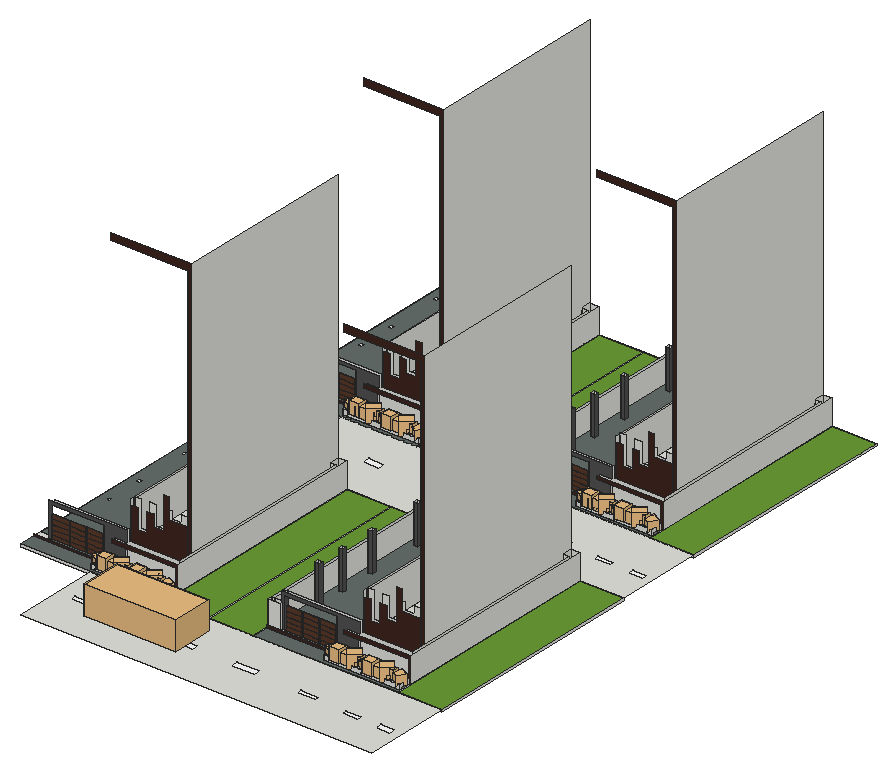
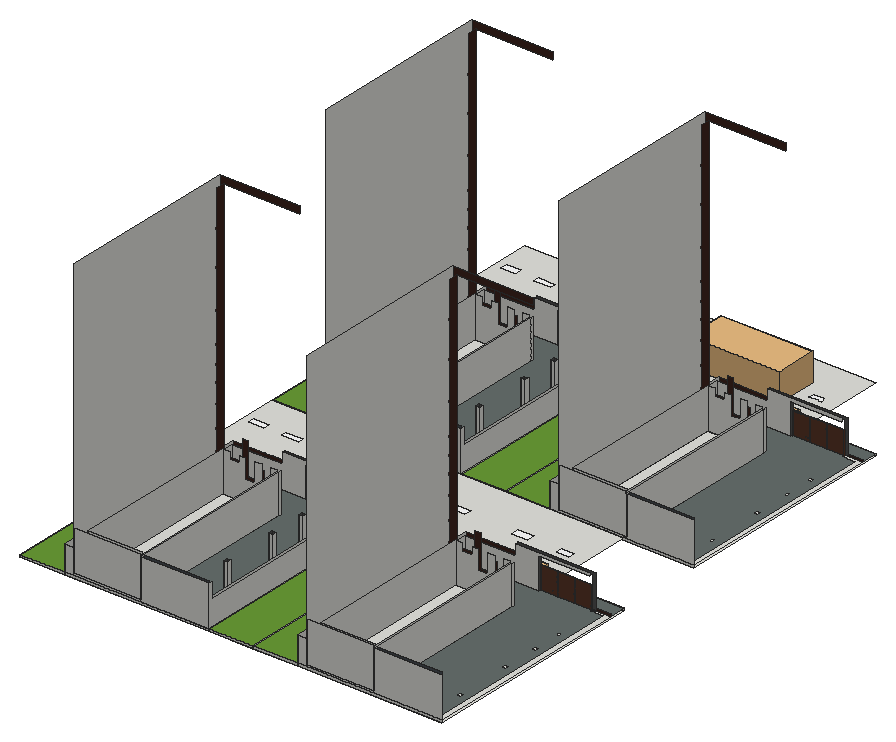
# SketchUp Ruby script. Lengths in inches.
U = 1.inch
M = Sketchup.active_model
def pt(a) = Geom::Point3d.new(a.map { |v| v * U })
def face(e, loops, mat)
  f = e.add_face(loops[0].map { |a| pt(a) })
  loops[1..].each { |l| e.add_face(l.map { |a| pt(a) }).erase! }
  f.material = f.back_material = mat if mat
  f
end
# faces: each face lists its corners as indices into pts; further lists are holes
def faces(e, pts, list, mat = nil) = list.each { |f| face(e, (f[0].is_a?(Array) ? f : [f]).map { |l| l.map { |i| pts[i] } }, mat) }
# xy, xz, yz: faces in a plane at the given z, y or x. An outline is a flat list of corners, or four numbers for a rectangle; further outlines are holes
def ring(l) = l.size == 4 ? [[l[0], l[1]], [l[2], l[1]], [l[2], l[3]], [l[0], l[3]]] : l.each_slice(2).to_a
def flat(e, list, mat, &to3) = list.each { |f| face(e, (f[0].is_a?(Array) ? f : [f]).map { |l| ring(l).map { |u, v| to3.(u, v) } }, mat) }
def xy(e, z, list, mat = nil) = flat(e, list, mat) { |x, y| [x, y, z] }
def xz(e, y, list, mat = nil) = flat(e, list, mat) { |x, z| [x, y, z] }
def yz(e, x, list, mat = nil) = flat(e, list, mat) { |y, z| [x, y, z] }
def lines(e, pts, list) = list.each { |a, b| e.add_line(pt(pts[a]), pt(pts[b])) }
# prism: a flat outline (further loops are holes) pulled along v
def prism(e, loops, v, mat = nil)
  f = face(e, loops, mat); d = Geom::Vector3d.new(v.map { |x| x * U })
  f.pushpull(f.normal.samedirection?(d) ? d.length : -d.length)
end
def box(e, o, s, mat = nil) = prism(e, [[o, [o[0] + s[0], o[1], o[2]], [o[0] + s[0], o[1] + s[1], o[2]], [o[0], o[1] + s[1], o[2]]]], [0, 0, s[2]], mat)
def at(x, y, z, deg = 0) = Geom::Transformation.translation(pt([x, y, z])) * Geom::Transformation.rotation(ORIGIN, Z_AXIS, deg.degrees)
def axes(o, x, y, z) = Geom::Transformation.new([*x, 0, *y, 0, *z, 0, *pt(o).to_a, 1])
def part(name) = M.definitions.add(name)
# library, detail: a bought-in or finely detailed component or shape, given as its bounding box
def library(name, o, s) = part(name).tap { |d| box(d.entities, o, s) }
def detail(e, o, s) = box(e.add_group.entities, o, s)
def put(e, d, t, mat = nil) = e.add_instance(d, t).tap { |i| i.material = mat if mat }
def group(e, t, mat = nil) = e.add_group.tap { |g| g.transformation = t; g.material = mat if mat }.entities
root = M.entities
M.materials.add("Color_").color = [255, 255, 255]
M.materials.add("Material__1").color = [95, 70, 46]
M.materials.add("[0043_SaddleBrown]").color = [63, 38, 31]
M.materials.add("[0135_DarkGray]").color = [81, 81, 81]
M.materials.add("[Color L16]").color = [51, 38, 20]
M.materials.add("[Formica Blue]").color = [73, 80, 86]
M.materials.add("[Grass Dark Green]").color = [105, 155, 54]
M.materials.add("[Slate]").color = [102, 110, 108]
M.materials.add("[Wood Veneer 01]").color = [89, 56, 41]
c1 = part("Grupo\#4")
xy(c1.entities,0,[[0,0,0,3.15,255.91,3.15,255.91,0,171.65,0,171.65,1.57,171.26,1.57,171.26,0,86.22,0,86.22,1.57,85.83,1.57,85.83,0]],"[Wood Veneer 01]")
xy(c1.entities,23.68,[[0,0,85.83,1.57],[86.22,0,171.26,1.57],[171.65,0,186.61,1.57],[186.61,0,255.91,1.57]],"[Color L16]")
xy(c1.entities,24.07,[[0,0,85.83,1.57],[86.22,0,168.11,1.57],[168.11,0,171.26,1.57],[171.65,0,255.91,1.57]],"[Color L16]")
xy(c1.entities,47.3,[[0,0,85.83,1.57],[86.22,0,89.76,1.57],[89.76,0,171.26,1.57],[171.65,0,255.91,1.57]],"[Color L16]")
xy(c1.entities,47.69,[[0,0,85.83,1.57],[86.22,0,171.26,1.57],[171.65,0,255.91,1.57]],"[Color L16]")
xy(c1.entities,70.92,[[0,0,85.83,1.57],[86.22,0,171.26,1.57],[171.65,0,255.91,1.57]],"[Color L16]")
xy(c1.entities,71.3125,[[0,0,85.83,1.57],[86.22,0,171.26,1.57],[171.65,0,255.91,1.57]],"[Color L16]")
xy(c1.entities,94.54,[[0,0,85.83,1.57],[86.22,0,171.26,1.57],[171.65,0,255.91,1.57]],"[Color L16]")
xy(c1.entities,94.9375,[[0,0,85.83,1.57],[86.22,0,171.26,1.57],[171.65,0,255.91,1.57]],"[Color L16]")
xy(c1.entities,118.16,[[0,0,85.83,0,85.83,1.57,86.22,1.57,86.22,0,171.26,0,171.26,1.57,171.65,1.57,171.65,0,255.91,0,255.91,3.15,0,3.15]],"[Wood Veneer 01]")
xz(c1.entities,0,[[0,0,85.83,23.68],[86.22,0,171.26,23.68],[171.65,0,255.91,23.68],[0,24.07,85.83,47.3],[86.22,24.07,171.26,47.3],
  [171.65,24.07,255.91,47.3],[0,47.69,85.83,70.92],[86.22,47.69,171.26,70.92],[171.65,47.69,255.91,70.92],[0,71.3125,85.83,94.54],
  [86.22,71.3125,171.26,94.54],[171.65,71.3125,255.91,94.54],[0,94.9375,85.83,118.16],[86.22,94.9375,171.26,118.16],[171.65,94.9375,255.91,118.16]],"[Wood Veneer 01]")
xz(c1.entities,1.57,[[[85.83,0,86.22,0,86.22,23.68,171.26,23.68,171.26,0,171.65,0,171.65,23.68,255.91,23.68,255.91,24.07,171.65,24.07,171.65,47.3,255.91,47.3,255.91,47.69,171.65,47.69,171.65,70.92,255.91,70.92,255.91,71.3125,171.65,71.3125,171.65,94.54,255.91,94.54,255.91,94.9375,171.65,94.9375,171.65,118.16,171.26,118.16,171.26,94.9375,86.22,94.9375,86.22,118.16,85.83,118.16,85.83,94.9375,0,94.9375,0,94.54,85.83,94.54,85.83,71.3125,0,71.3125,0,70.92,85.83,70.92,85.83,47.69,0,47.69,0,47.3,85.83,47.3,85.83,24.07,0,24.07,0,23.68,85.83,23.68],[86.22,71.3125,171.26,94.54],[86.22,24.07,171.26,47.3],[86.22,47.69,171.26,70.92]]],"[Color L16]")
xz(c1.entities,3.15,[[0,0,255.91,118.16]],"[Wood Veneer 01]")
yz(c1.entities,0,[[0,0,0,23.68,1.57,23.68,1.57,24.07,0,24.07,0,47.3,1.57,47.3,1.57,47.69,0,47.69,0,70.92,1.57,70.92,1.57,71.3125,0,71.3125,0,94.54,1.57,94.54,1.57,94.9375,0,94.9375,0,118.16,3.15,118.16,3.15,0]],"[Wood Veneer 01]")
yz(c1.entities,85.83,[[0,0,1.57,23.68],[0,24.07,1.57,47.3],[0,47.69,1.57,70.92],[0,71.3125,1.57,94.54],[0,94.9375,1.57,118.16]],"[Color L16]")
yz(c1.entities,86.22,[[0,0,1.57,23.68],[0,24.07,1.57,47.3],[0,47.69,1.57,70.92],[0,71.3125,1.57,94.54],[0,94.9375,1.57,118.16]],"[Color L16]")
yz(c1.entities,171.26,[[0,0,1.57,23.68],[0,24.07,1.57,47.3],[0,47.69,1.57,70.92],[0,71.3125,1.57,94.54],[0,94.9375,1.57,118.16]],"[Color L16]")
yz(c1.entities,171.65,[[0,0,1.57,23.68],[0,24.07,1.57,47.3],[0,47.69,1.57,70.92],[0,71.3125,1.57,94.54],[0,94.9375,1.57,118.16]],"[Color L16]")
yz(c1.entities,255.91,[[0,0,3.15,0,3.15,118.16,0,118.16,0,94.9375,1.57,94.9375,1.57,94.54,0,94.54,0,71.3125,1.57,71.3125,1.57,70.92,0,70.92,0,47.69,1.57,47.69,1.57,47.3,0,47.3,0,24.07,1.57,24.07,1.57,23.68,0,23.68]],"[Wood Veneer 01]")
c2 = library("Areca palm plant",[0,0,0],[49.1,36.6,54.46])
c3 = library("Group\#331",[-7.34,-1.2,0],[38.67,35.81,49.04])
c4 = library("Group38\#2",[14.01,28.44,-23.43],[18.58,18.32,38.89])
c5 = library("Group\#330",[-84.69,-90.07,-0.36],[176.51,175.13,171.4])
c6 = library("Group20\#1",[-20.81,-17.08,3.79],[39.86,39.43,37.51])
c7 = part("Group\#333")
put(c7.entities,c2,axes([-6.2,158.41,6.08],[0.45017,-0.56191,0],[0.66137,0.52986,0],[0,0,0.72]))
put(c7.entities,c2,axes([-6.2,56.6,6.08],[0.45017,-0.56191,0],[0.66137,0.52986,0],[0,0,0.72]))
put(c7.entities,c3,axes([24.9375,191.72,8],[0,0.79,0],[-0.79,0,0],[0,0,0.79]))
put(c7.entities,c4,axes([-4.1,100.66,28.17],[0.8848,0,0],[0,0.94674,0],[0,0,0.85826]))
g1 = group(c7.entities,at(0,0,0))
xy(g1,0,[[0,0,6,234.8],[30,0,36,234.8]])
xy(g1,3,[[6,0,30,234.8]])
xy(g1,7,[[6,5,30,229.8]],"Material__1")
xy(g1,15,[[[0,0,36,234.8],[6,5,30,229.8]]])
xz(g1,0,[[0,0,6,0,6,3,30,3,30,0,36,0,36,15,0,15]])
xz(g1,5,[[6,7,30,15]])
xz(g1,229.8,[[6,7,30,15]])
xz(g1,234.8,[[0,0,0,15,36,15,36,0,30,0,30,3,6,3,6,0]])
yz(g1,0,[[0,0,234.8,15]])
yz(g1,6,[[0,0,234.8,3],[5,7,229.8,15]])
yz(g1,30,[[0,0,234.8,3],[5,7,229.8,15]])
yz(g1,36,[[0,0,234.8,15]])
put(c7.entities,c5,axes([17.19,223.04,6.07],[-0.08133,-0.14087,0],[0.14087,-0.08133,0],[0,0,0.1725]))
put(c7.entities,c6,axes([18.97,181.79,4.77],[0,0.85,0],[-0.85,0,0],[0,0,0.85]))
put(c7.entities,c3,axes([24.9375,89.91,8],[0,0.79,0],[-0.79,0,0],[0,0,0.79]))
put(c7.entities,c4,axes([-4.1,-1.15,28.17],[0.8848,0,0],[0,0.94674,0],[0,0,0.85826]))
put(c7.entities,c5,axes([17.19,121.23,6.07],[-0.08133,-0.14087,0],[0.14087,-0.08133,0],[0,0,0.1725]))
put(c7.entities,c5,axes([14.93,91.37,6.05],[-0.04961,-0.08593,0],[0.08593,-0.04961,0],[0,0,0.10522]))
put(c7.entities,c5,axes([17.19,15.79,6.07],[-0.08133,-0.14087,0],[0.14087,-0.08133,0],[0,0,0.1725]))
put(c7.entities,c6,axes([18.97,79.98,4.77],[0,0.85,0],[-0.85,0,0],[0,0,0.85]))
put(c7.entities,c5,axes([14.93,44.05,6.05],[-0.04961,-0.08593,0],[0.08593,-0.04961,0],[0,0,0.10522]))
put(c7.entities,c5,axes([14.93,71.3,6.05],[-0.04961,-0.08593,0],[0.08593,-0.04961,0],[0,0,0.10522]))
put(c7.entities,c5,axes([14.93,173.12,6.05],[-0.04961,-0.08593,0],[0.08593,-0.04961,0],[0,0,0.10522]))
put(c7.entities,c5,axes([14.93,193.18,6.05],[-0.04961,-0.08593,0],[0.08593,-0.04961,0],[0,0,0.10522]))
put(c7.entities,c5,axes([14.93,145.87,6.05],[-0.04961,-0.08593,0],[0.08593,-0.04961,0],[0,0,0.10522]))
c8 = library("Group\#334",[0,0,0],[85.51,189.4,58.01])
c9 = part("2022 BMW i4")
put(c9.entities,c8,axes([0,0,0],[5,0,0],[0,5,0],[0,0,5]))
c10 = part("Untitled (5)")
xy(c10.entities,0,[[[158.81,26.5625,306.06,993.3125],[226.57,518.17,239.57,583.92],[225.28,357.51,237.28,411.51],[222.61,182.28,236.36,226.53],[239.71,931.55,251.46,972.3],[233.64,703.93,242.14,755.18],[240.05,835.03,248.8,880.53],[222.04,66.5,231.29,100.5]]])
xy(c10.entities,0,[[222.04,66.5,231.29,100.5],[222.61,182.28,236.36,226.53],[225.28,357.51,237.28,411.51],[226.57,518.17,239.57,583.92],[233.64,703.93,242.14,755.18],
  [240.05,835.03,248.8,880.53],[239.71,931.55,251.46,972.3]],"Color_")
xy(root,-7.1875,[[861.9375,272.41,1311.375,980.35],[1311.375,272.41,1448.875,980.35],[1448.875,272.41,1586.375,980.35],[1586.375,272.41,2035.8125,980.35],[2035.8125,272.41,2173.3125,980.35],
  [861.9375,1252.76,1311.375,1960.7],[1311.375,1252.76,1448.875,1960.7],[1448.875,1252.76,1586.375,1960.7],[1586.375,1252.76,2035.8125,1960.7],[2035.8125,1252.76,2173.3125,1960.7]])
xy(root,0,[[861.9375,324.35,1311.375,980.35],[1586.375,324.35,2035.8125,980.35],[861.9375,1304.7,1311.375,1960.7],[1586.375,1304.7,2035.8125,1960.7]])
xy(root,0,[[1311.375,272.41,1448.875,980.35],[1448.875,272.41,1586.375,980.35],[2035.8125,272.41,2173.3125,980.35],[1311.375,1252.76,1448.875,1960.7],[1448.875,1252.76,1586.375,1960.7],
  [2035.8125,1252.76,2173.3125,1960.7]],"[Grass Dark Green]")
xy(root,0,[[861.9375,272.41,1311.375,324.35],[1586.375,272.41,2035.8125,324.35],[861.9375,1252.76,1311.375,1304.7],[1586.375,1252.76,2035.8125,1304.7]],"[Slate]")
xy(root,6.125,[[1586.375,324.35,1626.62,328.54],[1626.62,324.35,1637.31,332.35],[1586.375,328.54,1626.62,343.16],[[1271.49,412.04,1271.49,438.72,1072.625,438.72,1072.625,980.35,1283.0625,980.35,1283.0625,412.04],[1078.41,447.84,1246.07,971.23]],[[1995.93,412.04,1995.93,438.72,1797.0625,438.72,1797.0625,980.35,2007.5,980.35,2007.5,412.04],[1802.84,447.84,1970.51,971.23]],
  [1078.41,447.84,1246.07,971.23],[1802.84,447.84,1970.51,971.23],[1615.83,475.13,1629.45,487.19],[1615.83,567.38,1629.45,579.44],[1615.83,682.44,1629.45,694.5],
  [1615.83,858.25,1629.45,870.31],[1586.375,1304.7,1626.62,1308.89],[1626.62,1304.7,1637.31,1312.7],[1586.375,1308.89,1626.62,1323.51],[[1271.49,1392.39,1271.49,1419.07,1072.625,1419.07,1072.625,1960.7,1283.0625,1960.7,1283.0625,1392.39],[1078.41,1428.19,1246.07,1951.58]],
  [[1995.93,1392.39,1995.93,1419.07,1797.0625,1419.07,1797.0625,1960.7,2007.5,1960.7,2007.5,1392.39],[1802.84,1428.19,1970.51,1951.58]],[1078.41,1428.19,1246.07,1951.58],[1802.84,1428.19,1970.51,1951.58],[1615.83,1455.48,1629.45,1467.54],[1615.83,1547.73,1629.45,1559.79],
  [1615.83,1662.79,1629.45,1674.85],[1615.83,1838.6,1629.45,1850.66]])
xy(root,6.125,[[[912.87,324.35,1072.88,324.35,1072.88,341.79,1301.69,341.79,1301.69,948.22,1283.0625,948.22,1283.0625,412.04,1271.49,412.04,1271.49,438.72,1072.625,438.72,1072.625,971.23,871.06,971.23,871.06,343.16,902.18,343.16,902.18,341.79,912.87,341.79],[891.39,858.25,905.02,870.31],[891.39,682.44,905.02,694.5],[891.39,567.38,905.02,579.44],[891.39,475.13,905.02,487.19]],[[1637.31,324.35,1797.32,324.35,1797.32,341.79,2026.13,341.79,2026.13,948.22,2007.5,948.22,2007.5,412.04,1995.93,412.04,1995.93,438.72,1797.0625,438.72,1797.0625,971.23,1595.49,971.23,1595.49,343.16,1626.62,343.16,1626.62,341.79,1637.31,341.79],[1615.83,858.25,1629.45,870.31],[1615.83,682.44,1629.45,694.5],[1615.83,567.38,1629.45,579.44],[1615.83,475.13,1629.45,487.19]],[[912.87,1304.7,1072.88,1304.7,1072.88,1322.14,1301.69,1322.14,1301.69,1928.57,1283.0625,1928.57,1283.0625,1392.39,1271.49,1392.39,1271.49,1419.07,1072.625,1419.07,1072.625,1951.58,871.06,1951.58,871.06,1323.51,902.18,1323.51,902.18,1322.14,912.87,1322.14],[891.39,1838.6,905.02,1850.66],[891.39,1662.79,905.02,1674.85],[891.39,1547.73,905.02,1559.79],[891.39,1455.48,905.02,1467.54]],[[1637.31,1304.7,1797.32,1304.7,1797.32,1322.14,2026.13,1322.14,2026.13,1928.57,2007.5,1928.57,2007.5,1392.39,1995.93,1392.39,1995.93,1419.07,1797.0625,1419.07,1797.0625,1951.58,1595.49,1951.58,1595.49,1323.51,1626.62,1323.51,1626.62,1322.14,1637.31,1322.14],[1615.83,1838.6,1629.45,1850.66],[1615.83,1662.79,1629.45,1674.85],[1615.83,1547.73,1629.45,1559.79],[1615.83,1455.48,1629.45,1467.54]]],"[Slate]")
xy(root,6.16,[[1072.88,324.35,1144.69,332.35],[1797.32,324.35,1869.13,332.35],[1072.88,1304.7,1144.69,1312.7],[1797.32,1304.7,1869.13,1312.7]])
xz(root,272.41,[[861.9375,-7.1875,1311.375,0],[1311.375,-7.1875,1448.875,0],[1448.875,-7.1875,1586.375,0],[1586.375,-7.1875,2035.8125,0],[2035.8125,-7.1875,2173.3125,0]])
xz(root,324.35,[[861.9375,0,1311.375,0,1311.375,77.97,1103.51,77.97,1103.51,67.07,1304.69,67.07,1304.69,14.13,1144.69,14.13,1144.69,6.16,1072.88,6.16,1072.88,6.125,861.9375,6.125],[1586.375,0,2035.8125,0,2035.8125,77.97,1827.94,77.97,1827.94,67.07,2029.13,67.07,2029.13,14.13,1869.13,14.13,1869.13,6.16,1797.32,6.16,1797.32,6.125,1586.375,6.125]],"[0043_SaddleBrown]")
xz(root,328.54,[[1586.375,6.125,1626.62,77.97]])
xz(root,332.35,[[902.18,6.125,912.87,6.125,912.87,102.02,1072.88,102.02,1072.88,6.16,1144.69,6.16,1144.69,67.07,1103.51,67.07,1103.51,77.97,1144.69,77.97,1144.69,111.97,902.18,111.97],[1626.62,6.125,1637.31,6.125,1637.31,102.02,1797.32,102.02,1797.32,6.16,1869.13,6.16,1869.13,67.07,1827.94,67.07,1827.94,77.97,1869.13,77.97,1869.13,111.97,1626.62,111.97]],"[0135_DarkGray]")
xz(root,341.79,[[1072.88,6.125,1072.88,102.02,912.87,102.02,912.87,111.97,1144.69,111.97,1144.69,77.97,1301.69,77.97,1301.69,6.125],[1626.62,6.125,1637.31,111.97],[1797.32,6.125,1797.32,102.02,1637.31,102.02,1637.31,111.97,1869.13,111.97,1869.13,77.97,2026.13,77.97,2026.13,6.125]])
xz(root,343.16,[[1586.375,6.125,1595.49,77.97],[1595.49,6.125,1626.62,77.97]])
xz(root,412.04,[[1271.49,6.125,1283.0625,6.125,1283.0625,866.5625,1033.03,866.5625,1033.03,845.41,1271.49,845.41],[1995.93,6.125,2007.5,6.125,2007.5,866.5625,1757.47,866.5625,1757.47,845.41,1995.93,845.41]],"[0043_SaddleBrown]")
xz(root,447.84,[[1078.41,6.125,1078.41,132.25,1094.98,132.25,1094.98,50.14,1123.6,50.14,1123.6,132.25,1144.2,132.25,1144.2,73.83,1175.45,73.83,1175.45,132.25,1191.74,132.25,1191.74,110.73,1224.86,110.73,1224.86,132.25,1246.07,132.25,1246.07,6.125],[1802.84,6.125,1802.84,132.25,1819.41,132.25,1819.41,50.14,1848.04,50.14,1848.04,132.25,1868.64,132.25,1868.64,73.83,1899.89,73.83,1899.89,132.25,1916.17,132.25,1916.17,110.73,1949.3,110.73,1949.3,132.25,1970.51,132.25,1970.51,6.125]])
xz(root,475.13,[[1615.83,6.125,1629.45,126.125]],"[0135_DarkGray]")
xz(root,487.19,[[1615.83,6.125,1629.45,126.125]])
xz(root,567.38,[[1615.83,6.125,1629.45,126.125]],"[0135_DarkGray]")
xz(root,579.44,[[1615.83,6.125,1629.45,126.125]])
xz(root,682.44,[[1615.83,6.125,1629.45,126.125]],"[0135_DarkGray]")
xz(root,694.5,[[1615.83,6.125,1629.45,126.125]])
xz(root,858.25,[[1615.83,6.125,1629.45,126.125]],"[0135_DarkGray]")
xz(root,870.31,[[1615.83,6.125,1629.45,126.125]])
xz(root,948.22,[[1283.0625,6.125,1301.69,77.97],[2007.5,6.125,2026.13,77.97]])
xz(root,971.23,[[1078.41,6.125,1246.07,132.25],[1802.84,6.125,1970.51,132.25]])
xz(root,971.23,[[871.06,6.125,1072.625,126.125],[1595.49,6.125,1797.0625,126.125]],"[Formica Blue]")
xz(root,980.35,[[861.9375,-7.1875,1311.375,0],[1311.375,-7.1875,1448.875,0],[1448.875,-7.1875,1586.375,0],[1586.375,-7.1875,2035.8125,0],[2035.8125,-7.1875,2173.3125,0],
  [861.9375,0,861.9375,126.125,1072.625,126.125,1072.625,6.125,1283.0625,6.125,1283.0625,77.97,1311.375,77.97,1311.375,0],[1586.375,0,1586.375,126.125,1797.0625,126.125,1797.0625,6.125,2007.5,6.125,2007.5,77.97,2035.8125,77.97,2035.8125,0],[1072.625,6.125,1072.625,126.125,1078.41,126.125,1078.41,132.25,1283.0625,132.25,1283.0625,6.125],[1797.0625,6.125,1797.0625,126.125,1802.84,126.125,1802.84,132.25,2007.5,132.25,2007.5,6.125]])
xz(root,1252.76,[[861.9375,-7.1875,1311.375,0],[1311.375,-7.1875,1448.875,0],[1448.875,-7.1875,1586.375,0],[1586.375,-7.1875,2035.8125,0],[2035.8125,-7.1875,2173.3125,0]])
xz(root,1304.7,[[861.9375,0,1311.375,0,1311.375,77.97,1103.51,77.97,1103.51,67.07,1304.69,67.07,1304.69,14.13,1144.69,14.13,1144.69,6.16,1072.88,6.16,1072.88,6.125,861.9375,6.125],[1586.375,0,2035.8125,0,2035.8125,77.97,1827.94,77.97,1827.94,67.07,2029.13,67.07,2029.13,14.13,1869.13,14.13,1869.13,6.16,1797.32,6.16,1797.32,6.125,1586.375,6.125]],"[0043_SaddleBrown]")
xz(root,1308.89,[[1586.375,6.125,1626.62,77.97]])
xz(root,1312.7,[[902.18,6.125,912.87,6.125,912.87,102.02,1072.88,102.02,1072.88,6.16,1144.69,6.16,1144.69,67.07,1103.51,67.07,1103.51,77.97,1144.69,77.97,1144.69,111.97,902.18,111.97],[1626.62,6.125,1637.31,6.125,1637.31,102.02,1797.32,102.02,1797.32,6.16,1869.13,6.16,1869.13,67.07,1827.94,67.07,1827.94,77.97,1869.13,77.97,1869.13,111.97,1626.62,111.97]],"[0135_DarkGray]")
xz(root,1322.14,[[1072.88,6.125,1072.88,102.02,912.87,102.02,912.87,111.97,1144.69,111.97,1144.69,77.97,1301.69,77.97,1301.69,6.125],[1626.62,6.125,1637.31,111.97],[1797.32,6.125,1797.32,102.02,1637.31,102.02,1637.31,111.97,1869.13,111.97,1869.13,77.97,2026.13,77.97,2026.13,6.125]])
xz(root,1323.51,[[1586.375,6.125,1595.49,77.97],[1595.49,6.125,1626.62,77.97]])
xz(root,1392.39,[[1271.49,6.125,1283.0625,6.125,1283.0625,866.5625,1033.03,866.5625,1033.03,845.41,1271.49,845.41],[1995.93,6.125,2007.5,6.125,2007.5,866.5625,1757.47,866.5625,1757.47,845.41,1995.93,845.41]],"[0043_SaddleBrown]")
xz(root,1428.19,[[1078.41,6.125,1078.41,132.25,1094.98,132.25,1094.98,50.14,1123.6,50.14,1123.6,132.25,1144.2,132.25,1144.2,73.83,1175.45,73.83,1175.45,132.25,1191.74,132.25,1191.74,110.73,1224.86,110.73,1224.86,132.25,1246.07,132.25,1246.07,6.125],[1802.84,6.125,1802.84,132.25,1819.41,132.25,1819.41,50.14,1848.04,50.14,1848.04,132.25,1868.64,132.25,1868.64,73.83,1899.89,73.83,1899.89,132.25,1916.17,132.25,1916.17,110.73,1949.3,110.73,1949.3,132.25,1970.51,132.25,1970.51,6.125]])
xz(root,1455.48,[[1615.83,6.125,1629.45,126.125]],"[0135_DarkGray]")
xz(root,1467.54,[[1615.83,6.125,1629.45,126.125]])
xz(root,1547.73,[[1615.83,6.125,1629.45,126.125]],"[0135_DarkGray]")
xz(root,1559.79,[[1615.83,6.125,1629.45,126.125]])
xz(root,1662.79,[[1615.83,6.125,1629.45,126.125]],"[0135_DarkGray]")
xz(root,1674.85,[[1615.83,6.125,1629.45,126.125]])
xz(root,1838.6,[[1615.83,6.125,1629.45,126.125]],"[0135_DarkGray]")
xz(root,1850.66,[[1615.83,6.125,1629.45,126.125]])
xz(root,1928.57,[[1283.0625,6.125,1301.69,77.97],[2007.5,6.125,2026.13,77.97]])
xz(root,1951.58,[[1078.41,6.125,1246.07,132.25],[1802.84,6.125,1970.51,132.25]])
xz(root,1951.58,[[871.06,6.125,1072.625,126.125],[1595.49,6.125,1797.0625,126.125]],"[Formica Blue]")
xz(root,1960.7,[[861.9375,-7.1875,1311.375,0],[1311.375,-7.1875,1448.875,0],[1448.875,-7.1875,1586.375,0],[1586.375,-7.1875,2035.8125,0],[2035.8125,-7.1875,2173.3125,0],
  [861.9375,0,861.9375,126.125,1072.625,126.125,1072.625,6.125,1283.0625,6.125,1283.0625,77.97,1311.375,77.97,1311.375,0],[1586.375,0,1586.375,126.125,1797.0625,126.125,1797.0625,6.125,2007.5,6.125,2007.5,77.97,2035.8125,77.97,2035.8125,0],[1072.625,6.125,1072.625,126.125,1078.41,126.125,1078.41,132.25,1283.0625,132.25,1283.0625,6.125],[1797.0625,6.125,1797.0625,126.125,1802.84,126.125,1802.84,132.25,2007.5,132.25,2007.5,6.125]])
yz(root,1072.625,[[438.72,6.125,438.72,109.76,441.04,109.76,441.04,112.41,438.72,112.41,438.72,126.125,447.84,126.125,447.84,6.125],[447.84,6.125,971.23,126.125],[971.23,6.125,980.35,126.125],[1419.07,6.125,1419.07,109.76,1421.39,109.76,1421.39,112.41,1419.07,112.41,1419.07,126.125,1428.19,126.125,1428.19,6.125],[1428.19,6.125,1951.58,126.125],
  [1951.58,6.125,1960.7,126.125]])
yz(root,1072.88,[[324.35,6.125,324.35,6.16,332.35,6.16,332.35,102.02,341.79,102.02,341.79,6.125],[1304.7,6.125,1304.7,6.16,1312.7,6.16,1312.7,102.02,1322.14,102.02,1322.14,6.125]],"[0135_DarkGray]")
yz(root,1078.41,[[447.84,6.125,971.23,126.125],[1428.19,6.125,1951.58,126.125]])
yz(root,1144.69,[[324.35,6.16,324.35,14.13,328.54,14.13,328.54,67.07,332.35,67.07,332.35,6.16],[1304.7,6.16,1304.7,14.13,1308.89,14.13,1308.89,67.07,1312.7,67.07,1312.7,6.16]])
yz(root,1246.07,[[447.84,6.125,971.23,132.25],[1428.19,6.125,1951.58,132.25]])
yz(root,1271.49,[[412.04,6.125,412.04,845.41,438.72,845.41,438.73,736,442.66,736,442.66,733.125,438.72,733.125,438.73,626.6,442.66,626.6,442.66,623.5625,438.73,623.5625,438.73,508.42,442.66,508.42,442.66,505.6875,438.73,505.6875,438.73,412.48,442.66,412.48,442.66,409.48,438.73,409.48,438.73,357.3,441.04,357.3,441.04,354.27,438.72,354.27,438.72,306.7,441.04,306.7,441.04,303,438.73,303,438.73,246.28,441.04,246.28,441.04,243.96,438.73,243.96,438.73,177.22,441.04,177.22,441.04,174.81,438.73,174.81,438.73,114.29,441.04,114.29,441.04,110.73,438.72,110.73,438.72,6.125],[1392.39,6.125,1392.39,845.41,1419.07,845.41,1419.08,736,1423.01,736,1423.01,733.125,1419.07,733.125,1419.08,626.6,1423.01,626.6,1423.01,623.5625,1419.08,623.5625,1419.08,508.42,1423.01,508.42,1423.01,505.6875,1419.08,505.6875,1419.08,412.48,1423.01,412.48,1423.01,409.48,1419.08,409.48,1419.08,357.3,1421.39,357.3,1421.39,354.27,1419.07,354.27,1419.07,306.7,1421.39,306.7,1421.39,303,1419.08,303,1419.08,246.28,1421.39,246.28,1421.39,243.96,1419.08,243.96,1419.08,177.22,1421.39,177.22,1421.39,174.81,1419.08,174.81,1419.08,114.29,1421.39,114.29,1421.39,110.73,1419.07,110.73,1419.07,6.125]],"[0043_SaddleBrown]")
yz(root,1283.0625,[[412.04,6.125,948.22,6.125,948.22,77.97,980.35,77.97,980.35,866.5625,412.04,866.5625],[948.22,6.125,980.35,77.97],[1392.39,6.125,1928.57,6.125,1928.57,77.97,1960.7,77.97,1960.7,866.5625,1392.39,866.5625],[1928.57,6.125,1960.7,77.97]])
yz(root,1301.69,[[341.79,6.125,948.22,77.97],[1322.14,6.125,1928.57,77.97]])
yz(root,1311.375,[[272.41,-7.1875,980.35,0],[1252.76,-7.1875,1960.7,0],[324.35,0,980.35,77.97],[1304.7,0,1960.7,77.97]])
yz(root,1448.875,[[272.41,-7.1875,980.35,0],[1252.76,-7.1875,1960.7,0]])
yz(root,1586.375,[[272.41,-7.1875,980.35,0],[1252.76,-7.1875,1960.7,0],[324.35,0,324.35,6.125,343.16,6.125,343.16,77.97,971.23,77.97,971.23,126.125,980.35,126.125,980.35,0],[1304.7,0,1304.7,6.125,1323.51,6.125,1323.51,77.97,1951.58,77.97,1951.58,126.125,1960.7,126.125,1960.7,0],[328.54,6.125,343.16,77.97],
  [1308.89,6.125,1323.51,77.97]])
yz(root,1595.49,[[343.16,6.125,971.23,77.97],[1323.51,6.125,1951.58,77.97]])
yz(root,1615.83,[[475.13,6.125,487.19,126.125],[567.38,6.125,579.44,126.125],[682.44,6.125,694.5,126.125],[858.25,6.125,870.31,126.125],[1455.48,6.125,1467.54,126.125],
  [1547.73,6.125,1559.79,126.125],[1662.79,6.125,1674.85,126.125],[1838.6,6.125,1850.66,126.125]])
yz(root,1626.62,[[328.54,6.125,332.35,77.97],[332.35,6.125,341.79,77.97],[341.79,6.125,343.16,77.97],[1308.89,6.125,1312.7,77.97],[1312.7,6.125,1322.14,77.97],
  [1322.14,6.125,1323.51,77.97]])
yz(root,1629.45,[[475.13,6.125,487.19,126.125],[567.38,6.125,579.44,126.125],[682.44,6.125,694.5,126.125],[858.25,6.125,870.31,126.125],[1455.48,6.125,1467.54,126.125],
  [1547.73,6.125,1559.79,126.125],[1662.79,6.125,1674.85,126.125],[1838.6,6.125,1850.66,126.125]],"[0135_DarkGray]")
yz(root,1637.31,[[332.35,6.125,341.79,102.02],[1312.7,6.125,1322.14,102.02]],"[0135_DarkGray]")
yz(root,1797.0625,[[438.72,6.125,438.72,109.76,441.04,109.76,441.04,112.41,438.72,112.41,438.72,126.125,447.84,126.125,447.84,6.125],[447.84,6.125,971.23,126.125],[971.23,6.125,980.35,126.125],[1419.07,6.125,1419.07,109.76,1421.39,109.76,1421.39,112.41,1419.07,112.41,1419.07,126.125,1428.19,126.125,1428.19,6.125],[1428.19,6.125,1951.58,126.125],
  [1951.58,6.125,1960.7,126.125]])
yz(root,1797.32,[[324.35,6.125,324.35,6.16,332.35,6.16,332.35,102.02,341.79,102.02,341.79,6.125],[1304.7,6.125,1304.7,6.16,1312.7,6.16,1312.7,102.02,1322.14,102.02,1322.14,6.125]],"[0135_DarkGray]")
yz(root,1802.84,[[447.84,6.125,971.23,126.125],[1428.19,6.125,1951.58,126.125]])
yz(root,1869.13,[[324.35,6.16,324.35,14.13,328.54,14.13,328.54,67.07,332.35,67.07,332.35,6.16],[1304.7,6.16,1304.7,14.13,1308.89,14.13,1308.89,67.07,1312.7,67.07,1312.7,6.16]])
yz(root,1970.51,[[447.84,6.125,971.23,132.25],[1428.19,6.125,1951.58,132.25]])
yz(root,1995.93,[[412.04,6.125,412.04,845.41,438.72,845.41,438.73,736,442.66,736,442.66,733.125,438.72,733.125,438.73,626.6,442.66,626.6,442.66,623.5625,438.73,623.5625,438.73,508.42,442.66,508.42,442.66,505.6875,438.73,505.6875,438.73,412.48,442.66,412.48,442.66,409.48,438.73,409.48,438.73,357.3,441.04,357.3,441.04,354.27,438.72,354.27,438.72,306.7,441.04,306.7,441.04,303,438.73,303,438.73,246.28,441.04,246.28,441.04,243.96,438.73,243.96,438.73,177.22,441.04,177.22,441.04,174.81,438.73,174.81,438.73,114.29,441.04,114.29,441.04,110.73,438.72,110.73,438.72,6.125],[1392.39,6.125,1392.39,845.41,1419.07,845.41,1419.08,736,1423.01,736,1423.01,733.125,1419.07,733.125,1419.08,626.6,1423.01,626.6,1423.01,623.5625,1419.08,623.5625,1419.08,508.42,1423.01,508.42,1423.01,505.6875,1419.08,505.6875,1419.08,412.48,1423.01,412.48,1423.01,409.48,1419.08,409.48,1419.08,357.3,1421.39,357.3,1421.39,354.27,1419.07,354.27,1419.07,306.7,1421.39,306.7,1421.39,303,1419.08,303,1419.08,246.28,1421.39,246.28,1421.39,243.96,1419.08,243.96,1419.08,177.22,1421.39,177.22,1421.39,174.81,1419.08,174.81,1419.08,114.29,1421.39,114.29,1421.39,110.73,1419.07,110.73,1419.07,6.125]],"[0043_SaddleBrown]")
yz(root,2007.5,[[412.04,6.125,948.22,6.125,948.22,77.97,980.35,77.97,980.35,866.5625,412.04,866.5625],[948.22,6.125,980.35,77.97],[1392.39,6.125,1928.57,6.125,1928.57,77.97,1960.7,77.97,1960.7,866.5625,1392.39,866.5625],[1928.57,6.125,1960.7,77.97]])
yz(root,2026.13,[[341.79,6.125,948.22,77.97],[1322.14,6.125,1928.57,77.97]])
yz(root,2035.8125,[[272.41,-7.1875,980.35,0],[1252.76,-7.1875,1960.7,0],[324.35,0,980.35,77.97],[1304.7,0,1960.7,77.97]])
yz(root,2173.3125,[[272.41,-7.1875,980.35,0],[1252.76,-7.1875,1960.7,0]])
p = [[1271.49,438.72,6.125],[1271.49,438.72,110.73],[1224.86,438.72,110.73],[1191.74,438.72,110.73],[1191.74,438.72,173.82],[1175.45,438.72,173.82],
  [1175.45,438.72,73.83],[1144.2,438.72,73.83],[1144.2,438.72,109.99],[1123.6,438.73,109.99],[1123.6,438.72,50.14],[1094.98,438.72,50.14],
  [1094.98,438.72,109.76],[1072.625,438.72,109.76],[1072.625,438.72,6.125],[1995.93,438.72,6.125],[1995.93,438.72,110.73],[1949.3,438.72,110.73],
  [1916.17,438.72,110.73],[1916.17,438.72,173.82],[1899.89,438.72,173.82],[1899.89,438.72,73.83],[1868.64,438.72,73.83],[1868.64,438.72,109.99],
  [1848.04,438.73,109.99],[1848.04,438.72,50.14],[1819.41,438.72,50.14],[1819.41,438.72,109.76],[1797.0625,438.72,109.76],[1797.0625,438.72,6.125],
  [1271.49,1419.07,6.125],[1271.49,1419.07,110.73],[1224.86,1419.07,110.73],[1191.74,1419.07,110.73],[1191.74,1419.07,173.82],[1175.45,1419.07,173.82],
  [1175.45,1419.07,73.83],[1144.2,1419.07,73.83],[1144.2,1419.07,109.99],[1123.6,1419.08,109.99],[1123.6,1419.07,50.14],[1094.98,1419.07,50.14],
  [1094.98,1419.08,109.76],[1072.625,1419.07,109.76],[1072.625,1419.07,6.125],[1995.93,1419.07,6.125],[1995.93,1419.07,110.73],[1949.3,1419.07,110.73],
  [1916.17,1419.07,110.73],[1916.17,1419.07,173.82],[1899.89,1419.07,173.82],[1899.89,1419.07,73.83],[1868.64,1419.07,73.83],[1868.64,1419.07,109.99],
  [1848.04,1419.08,109.99],[1848.04,1419.07,50.14],[1819.41,1419.07,50.14],[1819.41,1419.08,109.76],[1797.0625,1419.07,109.76],[1797.0625,1419.07,6.125]]
faces(root,p,[[0,1,2,3,4,5,6,7,8,9,10,11,12,13,14],[15,16,17,18,19,20,21,22,23,24,25,26,27,28,29],[30,31,32,33,34,35,36,37,38,39,40,41,42,43,44],[45,46,47,48,49,50,51,52,53,54,55,56,57,58,59]],"[0043_SaddleBrown]")
put(root,c1,axes([912.41,333.55,2.37],[0.6177,0,0],[0,0.6177,0],[0,0,0.6177]))
put(root,c1,axes([912.41,1313.9,2.37],[0.6177,0,0],[0,0.6177,0],[0,0,0.6177]))
put(root,c7,at(1307.32,284.24,0,90))
put(root,c7,at(1307.32,1264.59,0,90))
put(root,c9,axes([1203.68,221.46,0],[0,-0.3,0],[0.3,0,0],[0,0,0.3]))
put(root,c10,axes([1050.87,1546.56,0],[0,-1.85,0],[1.13,0,0],[0,0,1]))
put(root,c10,axes([1050.87,566.21,0],[0,-1.85,0],[1.13,0,0],[0,0,1]))
put(root,c1,axes([1636.85,333.55,2.37],[0.6177,0,0],[0,0.6177,0],[0,0,0.6177]))
put(root,c1,axes([1636.85,1313.9,2.37],[0.6177,0,0],[0,0.6177,0],[0,0,0.6177]))
put(root,c7,at(2031.75,1264.59,0,90))
put(root,c7,at(2031.75,284.24,0,90))
